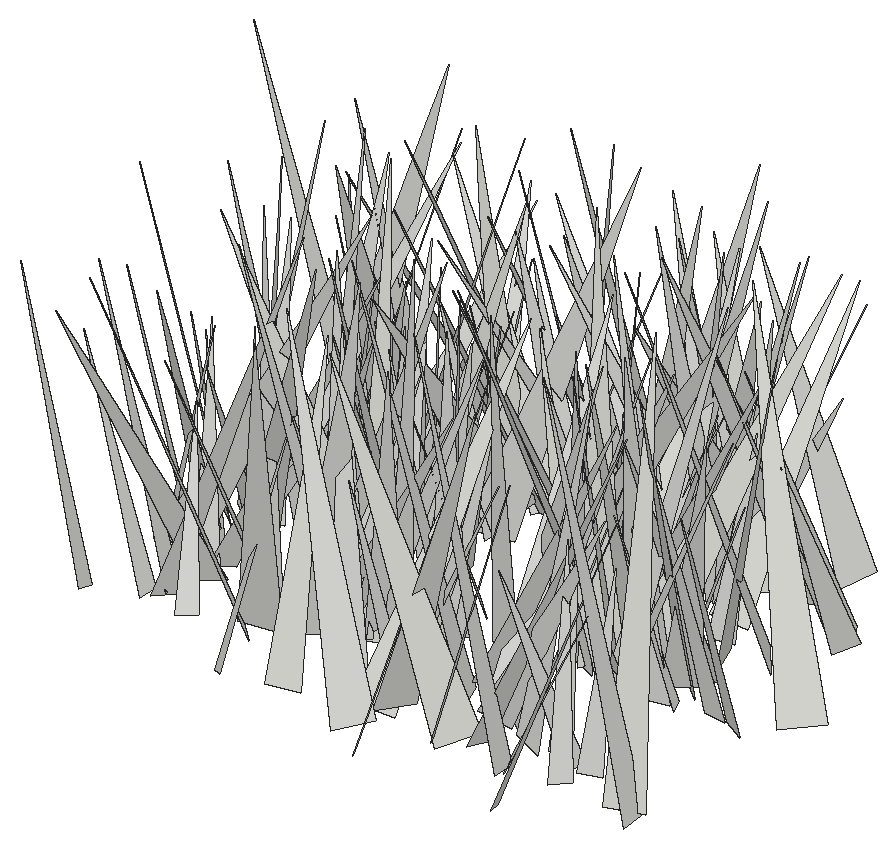
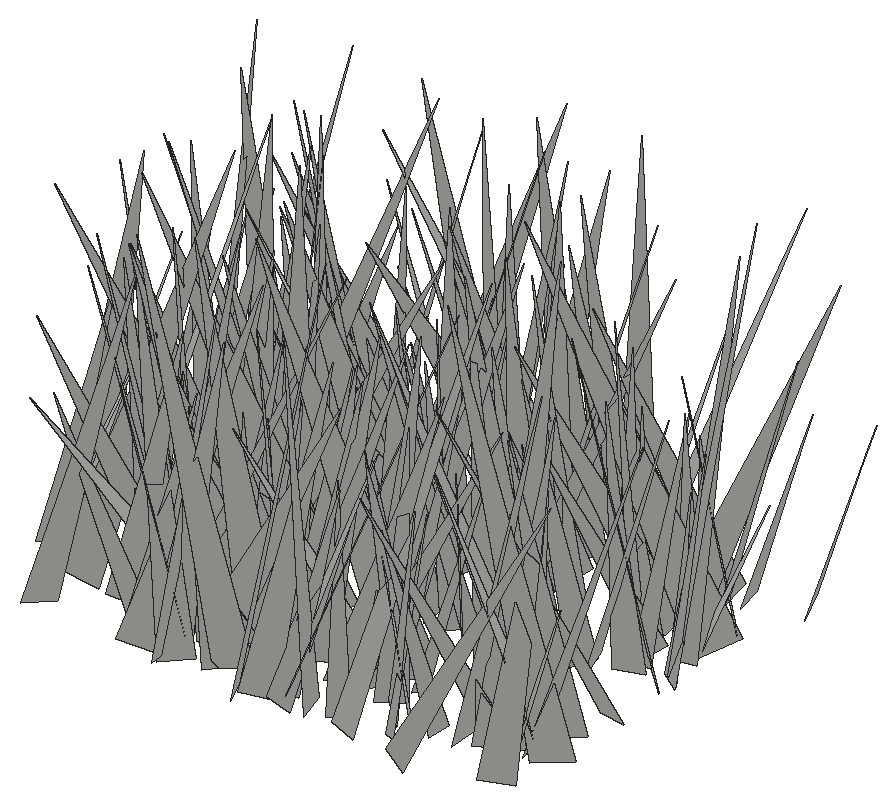
# SketchUp Ruby script. Lengths in inches.
U = 1.inch
M = Sketchup.active_model
def pt(a) = Geom::Point3d.new(a.map { |v| v * U })
def face(e, loops, mat)
  f = e.add_face(loops[0].map { |a| pt(a) })
  loops[1..].each { |l| e.add_face(l.map { |a| pt(a) }).erase! }
  f.material = f.back_material = mat if mat
  f
end
# faces: each face lists its corners as indices into pts; further lists are holes
def faces(e, pts, list, mat = nil) = list.each { |f| face(e, (f[0].is_a?(Array) ? f : [f]).map { |l| l.map { |i| pts[i] } }, mat) }
# xy, xz, yz: faces in a plane at the given z, y or x. An outline is a flat list of corners, or four numbers for a rectangle; further outlines are holes
def ring(l) = l.size == 4 ? [[l[0], l[1]], [l[2], l[1]], [l[2], l[3]], [l[0], l[3]]] : l.each_slice(2).to_a
def flat(e, list, mat, &to3) = list.each { |f| face(e, (f[0].is_a?(Array) ? f : [f]).map { |l| ring(l).map { |u, v| to3.(u, v) } }, mat) }
def xy(e, z, list, mat = nil) = flat(e, list, mat) { |x, y| [x, y, z] }
def xz(e, y, list, mat = nil) = flat(e, list, mat) { |x, z| [x, y, z] }
def yz(e, x, list, mat = nil) = flat(e, list, mat) { |y, z| [x, y, z] }
def lines(e, pts, list) = list.each { |a, b| e.add_line(pt(pts[a]), pt(pts[b])) }
# prism: a flat outline (further loops are holes) pulled along v
def prism(e, loops, v, mat = nil)
  f = face(e, loops, mat); d = Geom::Vector3d.new(v.map { |x| x * U })
  f.pushpull(f.normal.samedirection?(d) ? d.length : -d.length)
end
def box(e, o, s, mat = nil) = prism(e, [[o, [o[0] + s[0], o[1], o[2]], [o[0] + s[0], o[1] + s[1], o[2]], [o[0], o[1] + s[1], o[2]]]], [0, 0, s[2]], mat)
def at(x, y, z, deg = 0) = Geom::Transformation.translation(pt([x, y, z])) * Geom::Transformation.rotation(ORIGIN, Z_AXIS, deg.degrees)
def axes(o, x, y, z) = Geom::Transformation.new([*x, 0, *y, 0, *z, 0, *pt(o).to_a, 1])
def part(name) = M.definitions.add(name)
# library, detail: a bought-in or finely detailed component or shape, given as its bounding box
def library(name, o, s) = part(name).tap { |d| box(d.entities, o, s) }
def detail(e, o, s) = box(e.add_group.entities, o, s)
def put(e, d, t, mat = nil) = e.add_instance(d, t).tap { |i| i.material = mat if mat }
def group(e, t, mat = nil) = e.add_group.tap { |g| g.transformation = t; g.material = mat if mat }.entities
root = M.entities
c1 = part("fur_instance\#9")
p = [[0.8125,0,1.79],[0.67,-0.02,1.48],[0,-0.11,0],[0,0.11,0]]
faces(c1.entities,p,[[0,1,2,3]])
put(root,c1,axes([472.84,42.34,-21.86],[-5.74656,4.30747,2.03787],[4.75581,5.38477,2.02895],[0.29923,-2.86007,6.88916]))
put(root,c1,axes([476.6,39.5625,-21.86],[4.68389,2.5085,0.46697],[2.25732,-4.52881,1.68637],[-1.1896,1.28326,5.03861]))
put(root,c1,axes([475.14,42.1,-21.86],[3.88446,1.51086,0.00017],[1.46105,-3.75628,-1.06181],[0.38475,-0.98965,4.03042]))
put(root,c1,axes([469.49,40.97,-21.86],[-6.20404,3.776,0.73856],[3.82283,6.20814,0.37243],[0.43544,-0.70326,7.25325]))
put(root,c1,axes([469.79,42.79,-21.86],[6.355,-3.28716,0.66061],[-3.33311,-6.3472,0.48096],[-0.36352,0.73183,7.13864]))
put(root,c1,axes([462.65,43.82,-21.86],[-5.16383,-5.19186,0.43743],[-5.2089,5.15828,-0.26709],[0.11856,0.49863,7.31773]))
put(root,c1,axes([462.92,44.23,-21.86],[2.24537,-6.9608,0.71668],[-6.96969,-2.1575,0.8813],[0.62434,0.94895,7.26069]))
put(root,c1,axes([480.78,41.78,-21.86],[-7.60093,-1.69118,1.08047],[-1.85126,7.54274,-1.21718],[0.77483,1.43129,7.69108]))
put(root,c1,axes([477.04,43.34,-21.86],[0.84597,-3.78981,1.14812],[-3.67965,-1.18614,-1.20406],[-1.46323,0.79177,3.69169]))
put(root,c1,axes([471.96,42.2,-21.86],[4.69401,2.26049,0.88712],[2.32694,-4.7392,-0.23643],[-0.69438,-0.60059,5.20458]))
put(root,c1,axes([475.27,41.71,-21.86],[-7.26619,-2.16018,0.91047],[-2.32448,7.02333,-1.88745],[0.30351,2.07347,7.34176]))
put(root,c1,axes([470.62,39.66,-21.86],[6.47169,4.71895,0.84374],[4.29058,-6.33416,2.51645],[-2.13805,1.57262,7.60387]))
put(root,c1,axes([463.71,40.98,-21.86],[2.88186,3.44939,0.31018],[3.15851,-2.7832,1.60537],[-1.42067,0.8094,4.19835]))
put(root,c1,axes([477.31,42.17,-21.86],[-3.68366,1.92684,0.76086],[1.83141,3.75443,-0.64122],[0.96827,0.22919,4.10742]))
put(root,c1,axes([466.07,41.49,-21.86],[-1.14776,6.0133,0.84328],[6.0716,1.14805,0.07727],[0.08148,-0.84289,6.12137]))
put(root,c1,axes([459.61,45.74,-21.86],[0.6668,-6.36542,0.43774],[-6.10772,-0.7641,-1.80742],[-1.84553,0.22889,6.13974]))
put(root,c1,axes([477.73,43.23,-21.86],[-1.6026,3.32948,1.45838],[3.48573,1.8596,-0.41502],[1.03054,-1.11225,3.67172]))
put(root,c1,axes([472.91,44.2,-21.86],[2.62599,-5.06265,0.78885],[-4.77605,-2.09765,2.43674],[1.85526,1.76578,5.15641]))
put(root,c1,axes([468.62,44.36,-21.86],[-3.79793,-0.43925,1.06155],[-0.29859,3.91782,0.55288],[1.10936,-0.44932,3.78306]))
put(root,c1,axes([456.67,42.78,-21.86],[-5.41168,-1.42657,0.35166],[-1.45652,5.03228,-1.99993],[-0.1932,2.0214,5.22701]))
put(root,c1,axes([458.56,43.73,-21.86],[-4.63616,-0.58897,0.33378],[-0.62989,4.59941,-0.63319],[0.24806,0.67142,4.63033]))
put(root,c1,axes([475.93,43.92,-21.86],[-2.42915,2.39744,1.43013],[2.49267,2.71628,-0.31959],[1.25681,-0.75355,3.39799]))
put(root,c1,axes([473.52,42.63,-21.86],[6.28882,0.29269,0.74734],[0.08478,-6.11246,1.68051],[-0.79813,1.65699,6.06719]))
put(root,c1,axes([464.66,45.01,-21.86],[5.72788,-5.11466,1.67521],[-5.30647,-5.77538,0.51083],[-0.89854,1.50329,7.66207]))
put(root,c1,axes([466.98,43.83,-21.86],[1.5886,-5.12639,3.23902],[-5.9044,-2.07062,-0.3813],[-1.38174,2.95423,5.35333]))
put(root,c1,axes([460.48,43.38,-21.86],[-2.65941,2.49787,0.36396],[2.46932,2.68404,-0.37765],[0.52369,0.0288,3.62894]))
put(root,c1,axes([474.83,43.53,-21.86],[2.70818,5.99392,1.73773],[6.22026,-2.74585,-0.22279],[-0.5051,-1.67756,6.57356]))
put(root,c1,axes([480.12,42.08,-21.86],[-0.32528,8.12923,0.88129],[8.06717,0.17507,1.36272],[-1.33486,-0.92294,8.0208]))
put(root,c1,axes([461.41,46.38,-21.86],[-3.58338,-3.97137,0.418],[-3.89573,3.60001,0.80641],[0.87736,-0.23507,5.28792]))
put(root,c1,axes([466.74,46.08,-21.86],[2.07468,-5.92746,1.15005],[-6.03286,-1.98482,0.6533],[0.24901,1.299,6.24598]))
put(root,c1,axes([468.7,44.78,-21.86],[3.8277,2.64651,0.3376],[2.6435,-3.68235,-1.10521],[0.36045,-1.09797,4.52038]))
put(root,c1,axes([458.97,44.52,-21.86],[-5.59376,-1.56322,0.76508],[-1.67452,5.53596,-0.93185],[0.47433,1.10847,5.73284]))
put(root,c1,axes([471.3,44.89,-21.86],[-7.24522,-3.15461,1.03201],[-3.28219,7.17812,-1.10079],[0.49381,1.42581,7.82516]))
put(root,c1,axes([465.98,45.17,-21.86],[-6.93543,-2.32629,0.88421],[-2.41004,6.93097,-0.66862],[0.62063,0.91853,7.28456]))
put(root,c1,axes([467.8,45.45,-21.86],[-2.07525,-6.86081,3.30693],[-7.48887,2.46229,0.40886],[1.38687,3.02978,7.15613]))
put(root,c1,axes([464.85,45.8,-21.86],[4.53332,-3.78068,0.06575],[-3.6354,-4.32956,1.69931],[1.04008,1.34544,5.65304]))
put(root,c1,axes([457.58,48.37,-21.86],[-1.80775,-6.68688,0.47497],[-6.40102,1.86794,1.93536],[1.9917,-0.06601,6.65106]))
put(root,c1,axes([469.32,42.23,-21.86],[-4.67484,5.38464,0.57126],[4.73589,4.43174,-3.01759],[2.62527,1.59378,6.46085]))
put(root,c1,axes([457.66,45.52,-21.86],[3.51843,3.11531,1.14482],[3.25687,-3.56198,-0.31656],[-0.63919,-1.00114,4.68874]))
put(root,c1,axes([476.61,46.13,-21.86],[-3.5972,0.42819,0.55364],[0.48536,3.61469,0.35791],[0.50428,-0.42464,3.60487]))
put(root,c1,axes([459.07,43.98,-21.86],[6.5419,0.41912,1.71437],[-0.23349,-6.31856,2.43568],[-1.74935,2.41069,6.08602]))
put(root,c1,axes([464.67,46.52,-21.86],[-4.98307,4.13485,3.06586],[4.6284,5.46651,0.15019],[2.25263,-2.08511,6.47344]))
put(root,c1,axes([475.45,48.02,-21.86],[-4.28269,-7.03673,0.88853],[-7.06243,4.13524,-1.29164],[-0.65353,1.42504,8.13564]))
put(root,c1,axes([465.53,44.9375,-21.86],[1.79121,4.66243,0.42191],[4.67903,-1.79759,0.00003],[-0.15134,-0.39383,4.99466]))
put(root,c1,axes([465.98,46.38,-21.86],[3.63408,5.21962,1.38175],[5.32326,-3.18476,-1.96987],[0.90365,-2.23003,6.04736]))
put(root,c1,axes([465.93,48.52,-21.86],[-3.21608,-6.87634,1.40534],[-6.91778,3.36666,0.64196],[1.18463,0.99184,7.56406]))
put(root,c1,axes([461.64,45.5,-21.86],[-4.54245,-0.30979,1.16713],[-0.64985,4.4561,-1.34644],[1.01777,1.46262,4.34936]))
put(root,c1,axes([459.35,48.45,-21.86],[7.07591,-3.11018,0.05148],[-3.09924,-7.06002,-0.5432],[-0.26559,-0.47663,7.71016]))
put(root,c1,axes([459.13,46.125,-21.86],[-1.17354,4.22506,1.16991],[4.38332,1.15287,0.2334],[0.0799,-1.19029,4.3788]))
put(root,c1,axes([471.13,46.07,-21.86],[5.6454,-1.61471,0.55375],[-1.70236,-5.46688,1.41409],[-0.12614,1.5134,5.69896]))
put(root,c1,axes([470.58,48.1,-21.86],[5.01746,5.30698,2.27397],[5.71554,-4.13917,-2.95123],[0.81705,-3.63499,6.68051]))
put(root,c1,axes([468.27,47.51,-21.86],[4.61817,-3.87726,2.02523],[-4.05143,-4.90172,-0.14567],[-1.64942,1.18414,6.02822]))
put(root,c1,axes([476.12,50.36,-21.86],[-3.7888,-7.35051,1.42507],[-6.56657,4.02946,3.32556],[3.59735,-0.38635,7.57137]))
put(root,c1,axes([473.87,44.2,-21.86],[4.6203,4.92142,0.32663],[4.69042,-4.52255,1.79463],[-1.52544,1.00021,6.50745]))
put(root,c1,axes([475.52,47.16,-21.86],[5.31801,3.62577,0.57345],[3.65614,-5.14142,-1.39812],[0.32822,-1.47507,6.28273]))
put(root,c1,axes([457.16,49.66,-21.86],[-4.90749,-6.3294,1.61985],[-6.13533,5.16095,1.5783],[2.24565,0.26836,7.85199]))
put(root,c1,axes([479.5,48.63,-21.86],[-1.94034,-4.30134,0.80925],[-4.30819,2.03312,0.47669],[0.77193,0.53502,4.69459]))
put(root,c1,axes([463.92,46.3,-21.86],[6.69974,-1.69034,1.74311],[-2.11177,-6.58131,1.73465],[-1.19837,2.1474,6.68841]))
put(root,c1,axes([472.65,48.95,-21.86],[-1.45623,-6.82166,1.9418],[-6.84757,1.86878,1.42991],[1.84835,1.54881,6.82723]))
put(root,c1,axes([462.31,45.52,-21.86],[-6.71472,0.14595,1.05093],[-0.21339,6.41005,-2.25365],[1.03933,2.25902,6.32691]))
put(root,c1,axes([464.58,48.4,-21.86],[-7.38136,0.22251,0.33251],[0.26326,7.32737,0.9407],[0.30128,-0.95116,7.32455]))
put(root,c1,axes([458.59,49.45,-21.86],[-0.44013,-4.40012,0.04518],[-4.35564,0.44209,0.62427],[0.62566,-0.01764,4.37779]))
put(root,c1,axes([470.26,48.11,-21.86],[-1.72933,-6.01967,2.37326],[-6.41752,1.90965,0.16749],[0.82719,2.23073,6.26091]))
put(root,c1,axes([457.25,46.99,-21.86],[6.5519,-4.81181,0.9912],[-4.80718,-5.93833,2.94799],[1.01342,2.94042,7.57563]))
put(root,c1,axes([474.39,48.88,-21.86],[4.90048,2.76624,3.25214],[3.64641,-5.28694,-0.99757],[-2.22086,-2.5767,5.5382]))
put(root,c1,axes([466.49,46.08,-21.86],[-5.1152,1.11044,1.16629],[0.73583,5.06638,-1.59654],[1.43244,1.36283,4.98492]))
put(root,c1,axes([468.25,47.1,-21.86],[1.29664,4.3065,0.97913],[4.41517,-1.23995,-0.39328],[0.1042,-1.05001,4.48024]))
put(root,c1,axes([467.59,47.84,-21.86],[-4.97388,0.03891,0.99351],[0.0174,5.07103,-0.11152],[0.99411,0.10595,4.97278]))
put(root,c1,axes([467.87,49.89,-21.86],[-3.10311,-4.08719,0.56583],[-3.96021,3.14894,1.02739],[1.15846,-0.18348,5.02781]))
put(root,c1,axes([478.54,48.85,-21.86],[-1.41742,-4.71426,1.18858],[-4.85717,1.31918,-0.56008],[-0.21176,1.29675,4.89077]))
put(root,c1,axes([472.74,47.15,-21.86],[3.10796,2.24348,0.34109],[2.21254,-3.12436,0.38987],[-0.50422,0.11876,3.81322]))
put(root,c1,axes([474.71,49.58,-21.86],[-2.15861,-6.19615,1.53511],[-6.31129,2.3146,0.46773],[0.95736,1.28794,6.5447]))
put(root,c1,axes([457.85,47.08,-21.86],[-4.45593,-2.02584,0.38216],[-1.95722,3.87117,-2.29973],[-0.64758,2.23951,4.32095]))
put(root,c1,axes([463.16,51.05,-21.86],[-1.84691,-6.18778,0.26193],[-5.9057,1.84189,1.87043],[1.86547,-0.29517,6.18071]))
put(root,c1,axes([472.33,45.86,-21.86],[-2.04424,6.85145,0.72305],[6.79433,2.1298,-0.97223],[1.1412,-0.40704,7.08351]))
put(root,c1,axes([476.36,49.76,-21.86],[4.15858,-4.6502,0.45845],[-4.67236,-4.14601,0.32855],[-0.05962,0.56087,6.22978]))
put(root,c1,axes([477.08,48.64,-21.86],[-3.24657,-1.58505,0.39086],[-1.61743,3.24104,-0.29141],[0.22149,0.43432,3.60107]))
put(root,c1,axes([458.31,47.83,-21.86],[1.10778,3.32388,1.25845],[3.28018,-1.46364,0.97838],[-1.36832,-0.8177,3.36424]))
put(root,c1,axes([466.34,45.76,-21.86],[0.27633,8.1596,0.76138],[7.93766,-0.45592,2.00518],[-2.0377,-0.66947,7.91421]))
put(root,c1,axes([459.36,46.67,-21.86],[6.04009,-0.71684,0.90558],[-1.00409,-5.64184,2.23115],[-0.57074,2.3393,5.65849]))
put(root,c1,axes([467.11,48.35,-21.86],[3.97041,-1.42005,1.05601],[-1.57618,-4.01704,0.5243],[-0.80459,0.86179,4.18399]))
put(root,c1,axes([474.36,50.43,-21.86],[3.11086,-6.46121,1.0779],[-6.53922,-3.13316,0.09147],[-0.38422,1.01124,7.17051]))
put(root,c1,axes([476.76,50.81,-21.86],[-0.49515,-5.81147,0.35136],[-5.82208,0.49376,-0.03799],[-0.0081,0.35331,5.8324]))
put(root,c1,axes([476.39,48.49,-21.86],[-0.90978,-4.59674,2.27002],[-5.08569,0.51819,-0.98893],[-0.64715,2.39002,4.58036]))
put(root,c1,axes([458.76,48.4,-21.86],[3.29977,-2.51906,0.3221],[-2.3698,-2.86445,1.87534],[0.91296,1.66948,3.70368]))
put(root,c1,axes([457.1,49.63,-21.86],[-2.14945,-3.42966,1.0737],[-3.50191,2.27993,0.27214],[0.80747,0.75821,4.03839]))
put(root,c1,axes([465.57,47.7,-21.86],[-4.06355,5.05875,1.67662],[5.05755,4.32523,-0.79246],[1.68023,-0.78477,6.44014]))
put(root,c1,axes([475.32,47.42,-21.86],[2.96798,6.81466,1.03357],[6.887,-2.97737,-0.1458],[-0.27767,-1.00619,7.4315]))
put(root,c1,axes([463.35,46.91,-21.86],[2.8075,7.47142,1.47372],[7.21104,-3.11318,2.04573],[-2.44844,-0.60171,7.71486]))
put(root,c1,axes([459.7,48.22,-21.86],[-6.13991,-1.94187,2.86824],[-2.65031,6.39227,-1.34568],[2.23013,2.25037,6.2975]))
put(root,c1,axes([460.17,50.5,-21.86],[4.67852,-1.7119,0.20248],[-1.71617,-4.68064,0.08066],[-0.16239,0.14538,4.98123]))
put(root,c1,axes([473.03,50.95,-21.86],[-3.56669,-5.90918,0.59479],[-5.71236,3.22345,-2.22975],[-1.62517,1.63841,6.53207]))
put(root,c1,axes([466.43,50.08,-21.86],[4.38059,2.58911,2.20412],[2.75267,-4.81057,0.18002],[-1.99611,-0.9519,5.08534]))
put(root,c1,axes([473.29,49.41,-21.86],[-7.16118,3.19135,1.99245],[3.1192,7.43157,-0.69239],[2.1036,-0.15533,7.80947]))
put(root,c1,axes([458.63,49.99,-21.86],[-1.35199,5.16754,1.66066],[5.39955,1.4549,-0.13134],[0.55327,-1.57128,5.33986]))
put(root,c1,axes([466.04,51.18,-21.86],[5.32416,0.8497,1.29821],[1.01973,-5.41351,-0.63884],[-1.1694,-0.85204,5.35356]))
put(root,c1,axes([462.61,52.26,-21.86],[4.90607,-3.46037,0.24315],[-3.44997,-4.91123,-0.28332],[-0.36191,-0.09172,5.99695]))
put(root,c1,axes([464.875,51.35,-21.86],[2.7967,-3.72992,1.22325],[-3.91864,-2.74089,0.60164],[-0.23004,1.34365,4.62297]))
put(root,c1,axes([477.53,53.06,-21.86],[-6.16047,-5.25921,0.96963],[-5.25018,6.22911,0.42963],[1.01736,0.29959,8.08864]))
put(root,c1,axes([459.83,50.47,-21.86],[-6.22819,-1.34042,0.61243],[-1.44458,6.07908,-1.38568],[0.29149,1.48668,6.21828]))
put(root,c1,axes([469.69,54.03,-21.86],[-1.30326,-6.4856,0.41929],[-6.05179,1.36694,2.33336],[2.36951,-0.07596,6.19006]))
put(root,c1,axes([464.85,55.5,-21.86],[6.08431,-4.17162,0.61258],[-3.3903,-5.47976,-3.64343],[-2.50671,-2.71408,6.41457]))
put(root,c1,axes([481.18,50.18,-21.86],[-5.24663,5.623,0.95369],[5.70188,5.20042,0.70642],[0.12741,-1.17997,7.65808]))
put(root,c1,axes([457.58,49.91,-21.86],[4.64173,5.41011,1.53464],[5.42173,-4.8336,0.64123],[-1.49305,-0.73288,7.09956]))
put(root,c1,axes([474.84,52.28,-21.86],[3.70621,1.73352,0.50221],[1.78343,-3.34171,-1.62653],[0.27688,-1.67963,3.75439]))
put(root,c1,axes([461.38,50.32,-21.86],[-4.14484,-0.82966,2.07391],[-1.4546,4.32013,-1.17886],[1.69516,1.67847,4.05935]))
put(root,c1,axes([476.33,52.06,-21.86],[6.26752,1.77798,1.53658],[2.00319,-6.33057,-0.84565],[-1.22862,-1.25168,6.45971]))
put(root,c1,axes([469.45,52.57,-21.86],[3.81653,-4.78014,0.36891],[-4.62204,-3.54318,1.90641],[1.2738,1.46558,5.81217]))
put(root,c1,axes([470.42,51.53,-21.86],[-1.43576,4.62376,1.24523],[4.74317,1.1948,1.0324],[-0.65727,-1.47798,4.73019]))
put(root,c1,axes([472.49,52.375,-21.86],[5.56558,-2.4926,0.3103],[-2.49513,-5.39934,1.38077],[0.28926,1.38533,5.93988]))
put(root,c1,axes([469.34,54.14,-21.86],[-3.93498,0.71077,2.15609],[1.47172,4.08376,1.33974],[1.72857,-1.85895,3.76754]))
put(root,c1,axes([468.71,53.08,-21.86],[6.17977,-5.38552,0.13557],[-5.06059,-5.73249,2.95646],[1.84733,2.31224,7.64543]))
put(root,c1,axes([463.34,52.11,-21.86],[2.20928,6.37096,1.50715],[6.50914,-1.9672,-1.22586],[0.70121,-1.81177,6.63078]))
put(root,c1,axes([470.39,54.03,-21.86],[0.55845,-3.67703,0.59896],[-3.72525,-0.55803,0.04757],[-0.0423,0.59936,3.71889]))
put(root,c1,axes([475.46,53.04,-21.86],[-1.45732,3.49071,1.72371],[3.67662,1.83923,-0.61623],[1.28012,-1.30851,3.73217]))
put(root,c1,axes([474.17,51.19,-21.86],[-6.70082,0.16595,0.10129],[0.12128,6.29761,-2.29436],[0.15195,2.29157,6.29797]))
put(root,c1,axes([458.85,56.79,-21.86],[7.11754,-4.23376,0.53848],[-3.90576,-6.88369,-2.49681],[-1.7204,-1.88792,7.89621]))
put(root,c1,axes([473.84,51.23,-21.86],[-0.75445,7.6495,1.46212],[7.18414,1.25072,-2.83648],[3.00677,-1.06897,7.14412]))
put(root,c1,axes([465.08,54.12,-21.86],[-4.43499,0.78648,1.49873],[1.10021,4.53377,0.87655],[1.28619,-1.16631,4.41807]))
put(root,c1,axes([472.4375,52.11,-21.86],[-1.23415,4.06964,0.18802],[4.01431,1.18128,0.78126],[-0.69473,-0.40381,4.18028]))
put(root,c1,axes([479.04,55.21,-21.86],[3.36953,-3.09183,0.80409],[-2.80421,-3.42236,-1.4084],[-1.53048,-0.53643,4.35081]))
put(root,c1,axes([462.41,51.5,-21.86],[6.70956,3.50603,1.11128],[3.28027,-6.75003,1.49074],[-1.66343,0.8308,7.42214]))
put(root,c1,axes([478.33,55.42,-21.86],[-4.87517,-3.87645,0.62854],[-3.83008,4.91477,0.6039],[0.86741,-0.08574,6.19915]))
put(root,c1,axes([460.75,54.97,-21.86],[3.22144,-2.0672,0.86258],[-1.86043,-3.31076,-0.98626],[-1.24746,-0.40075,3.69841]))
put(root,c1,axes([472.48,52.91,-21.86],[3.75823,0.40452,0.85087],[0.18545,-3.74836,0.96295],[-0.9237,0.89332,3.65522]))
put(root,c1,axes([472.27,53.09,-21.86],[-3.57041,1.71359,0.7726],[1.61509,3.64514,-0.62093],[0.96166,0.24019,3.91135]))
put(root,c1,axes([476.71,56.74,-21.66],[0.82289,-7.98079,0.80674],[-7.83354,-0.97405,-1.64552],[-1.72608,0.61581,7.85254]))
put(root,c1,axes([463.17,55.43,-21.86],[-3.68775,-0.43694,1.2324],[0.03671,3.65173,1.40455],[1.30705,-1.33536,3.43768]))
put(root,c1,axes([470.85,53.98,-21.86],[3.29309,2.39527,0.08068],[2.3726,-3.23886,-0.68467],[0.3385,-0.60058,4.0141]))
put(root,c1,axes([472.77,56.27,-21.66],[-6.88482,-1.0416,0.48285],[-0.90858,6.73783,1.57954],[0.70182,-1.49517,6.78165]))
put(root,c1,axes([459.96,53.21,-21.86],[-5.24858,-0.93793,1.2858],[-1.33069,5.01688,-1.77222],[0.87308,2.00792,5.02857]))
put(root,c1,axes([464.95,53.86,-21.86],[5.54256,-5.39998,2.31392],[-5.86744,-4.92827,2.55329],[0.29519,3.43313,7.30483]))
put(root,c1,axes([468.37,54.75,-21.86],[-4.97411,1.9133,1.24146],[2.05101,5.05519,0.42681],[0.99764,-0.85328,5.31228]))
put(root,c1,axes([466.625,58.12,-21.86],[-5.86145,-3.99032,0.23805],[-3.68658,5.55942,2.41617],[1.54546,-1.87245,6.66644]))
put(root,c1,axes([467.24,55.92,-21.86],[3.86572,-4.28586,2.24353],[-4.19582,-4.39988,-1.17556],[-2.40771,0.7863,5.6507]))
put(root,c1,axes([473.4375,55.6,-21.86],[-6.84332,-0.22544,2.15666],[-0.013,7.14388,0.70553],[2.16837,-0.66867,6.81058]))
put(root,c1,axes([457.0625,52.83,-21.86],[2.4491,6.4359,0.09226],[6.32974,-2.3903,-1.28384],[1.16776,-0.54137,6.7654]))
put(root,c1,axes([470.93,52.76,-21.86],[-1.68385,4.77561,0.18208],[4.53538,1.65768,-1.53538],[1.50664,0.34725,4.82539]))
put(root,c1,axes([461.58,55.07,-21.86],[3.09242,2.58599,1.68004],[2.84079,-3.31463,-0.12697],[-1.19992,-1.18273,4.02918]))
put(root,c1,axes([458.24,56.45,-21.86],[-0.42992,-4.68733,0.89248],[-4.33891,0.75688,1.88505],[1.98531,0.63912,4.31306]))
put(root,c1,axes([474.08,55.64,-21.86],[4.94298,-3.20176,1.42299],[-3.34359,-5.04595,0.26096],[-1.0472,0.99819,5.88356]))
put(root,c1,axes([465.36,56.08,-21.86],[-3.41079,-4.86692,0.40111],[-4.72199,3.16213,-1.78467],[-1.24525,1.33989,5.66881]))
put(root,c1,axes([473.08,52.46,-21.86],[-5.5806,3.5391,0.90465],[3.04631,5.42049,-2.4135],[2.01583,1.60617,6.15169]))
put(root,c1,axes([457.4,54.7,-21.86],[2.82826,-4.43632,2.67471],[-5.15951,-2.68482,1.00262],[-0.46309,2.81866,5.16476]))
put(root,c1,axes([478.62,56.17,-21.86],[-4.47388,-2.50611,0.21033],[-2.51468,4.46372,-0.30343],[0.03476,0.36756,5.119]))
put(root,c1,axes([468.42,55.99,-21.86],[-4.16703,-2.76107,2.92288],[-2.78486,5.0182,0.77013],[2.90022,0.85149,4.93909]))
put(root,c1,axes([472.5,58.83,-21.86],[3.62515,-5.36286,0.15908],[-5.03579,-3.46731,-2.13211],[-1.85105,-1.06996,6.11196]))
put(root,c1,axes([469.62,55.74,-21.86],[6.54433,-2.87567,1.841],[-3.10892,-6.66403,0.64215],[-1.41189,1.3447,7.11937]))
put(root,c1,axes([473.12,55.3,-21.86],[3.79421,5.57197,1.64798],[5.81056,-3.63804,-1.07735],[0.00109,-1.96889,6.65448]))
put(root,c1,axes([463.58,59.05,-21.86],[-3.81436,-7.20009,0.2192],[-7.12697,3.80817,1.069],[1.0467,-0.30859,8.07762]))
put(root,c1,axes([464.49,55.94,-21.86],[-6.37075,2.32719,2.17346],[2.54476,6.64308,0.34616],[1.91413,-1.08621,6.77365]))
put(root,c1,axes([471.48,54.61,-21.86],[7.05742,-1.09775,2.22467],[-1.64487,-7.09246,1.71837],[-1.85705,2.1103,6.93249]))
put(root,c1,axes([467.2,53.7,-21.86],[4.59925,2.87418,0.36346],[2.61006,-4.40682,1.82035],[-1.25721,1.36572,5.10885]))
put(root,c1,axes([457.16,58.87,-21.66],[4.65411,-4.15615,0.09318],[-4.0063,-4.52139,-1.56511],[-1.10988,-1.10744,6.04026]))
put(root,c1,axes([470.58,57.67,-21.66],[4.65665,4.64477,2.8893],[5.46904,-4.02795,-2.33914],[-0.10763,-3.71592,6.14709]))
put(root,c1,axes([460.09,56.95,-21.86],[-6.59248,-1.12335,1.64682],[-1.04061,6.79216,0.46743],[1.70031,-0.1986,6.67115]))
put(root,c1,axes([458.04,55.73,-21.86],[-7.51977,-1.08655,0.44758],[-1.14316,7.43533,-1.15625],[0.27218,1.20961,7.50937]))
put(root,c1,axes([456.54,56.65,-21.66],[0.11593,7.32982,3.76994],[7.80213,1.11829,-2.4142],[2.6581,-3.60212,6.9218]))
put(root,c1,axes([465.49,56.51,-21.86],[-4.72001,4.32069,1.36462],[4.52973,4.45158,1.57294],[-0.11027,-2.07946,6.20264]))
put(root,c1,axes([463.49,56.55,-21.86],[2.88206,-3.90926,2.29022],[-4.22914,-3.29495,-0.30223],[-1.62535,1.64154,4.8474]))
put(root,c1,axes([466.43,58.97,-21.86],[-1.51656,-6.50321,0.08888],[-6.50028,1.51258,-0.24097],[-0.21452,0.14123,6.67335]))
put(root,c1,axes([469.66,56.38,-21.86],[3.69637,0.13401,0.11411],[0.12786,-3.69317,0.19555],[-0.12096,0.19138,3.69362]))
put(root,c1,axes([474.82,54.26,-21.86],[-1.93845,6.02083,0.54238],[5.77969,2.01278,-1.68701],[1.77192,0.02133,6.09606]))
put(root,c1,axes([472.61,56.125,-21.86],[4.17066,5.06918,1.33611],[5.23853,-4.09478,-0.81653],[-0.19883,-1.55319,6.51339]))
put(root,c1,axes([463.98,54.93,-21.86],[-3.2921,4.67046,0.35788],[4.62081,3.30978,-0.68745],[0.76768,0.10645,5.67261]))
put(root,c1,axes([470.97,56.27,-21.86],[-3.29072,5.65648,0.59206],[5.32719,2.82602,2.60955],[-1.99181,-1.7869,6.00123]))
put(root,c1,axes([470.85,58.76,-21.86],[1.7793,-6.50243,0.4842],[-6.28195,-1.575,1.93351],[1.74732,0.95904,6.45825]))
put(root,c1,axes([462.09,58.41,-21.86],[-2.01295,-3.23513,0.63988],[-3.06607,2.112,1.03257],[1.21439,-0.03018,3.66768]))
put(root,c1,axes([469.43,58.34,-21.86],[2.01974,-4.62687,0.27657],[-4.52399,-1.90214,1.21619],[1.00891,0.73329,4.89981]))
put(root,c1,axes([461.68,57.7,-21.86],[4.05743,2.55482,1.17911],[2.80714,-3.81746,-1.3882],[-0.19333,-1.81108,4.58942]))
put(root,c1,axes([473.25,57.9375,-21.86],[3.41803,-2.18502,2.15563],[-1.95303,-4.03718,-0.99543],[-2.36786,0.1758,3.93273]))
put(root,c1,axes([464.22,58.4375,-21.86],[1.68223,-3.64936,0.16027],[-3.63941,-1.65928,0.41825],[0.31341,0.31999,3.9966]))
put(root,c1,axes([467.22,59.01,-21.86],[2.93992,-5.13493,1.13143],[-5.01799,-3.12719,-1.15379],[-1.5708,0.37938,5.8034]))
put(root,c1,axes([458.1,56.64,-21.66],[-3.16034,-1.96863,0.75138],[-2.10046,2.8354,-1.40585],[-0.16774,1.5852,3.44773]))
put(root,c1,axes([474.65,56.7,-21.86],[-2.33709,5.71521,1.48586],[5.84354,2.00796,1.46781],[-0.85111,-1.90732,5.99759]))
put(root,c1,axes([461.02,57.1,-21.86],[3.85375,-0.57416,0.66525],[-0.65849,-3.86826,0.47595],[-0.58191,0.57487,3.8671]))
put(root,c1,axes([466.5625,58.24,-21.86],[0.87067,-3.63818,0.96208],[-3.64876,-1.05785,-0.69825],[-0.92116,0.75142,3.67517]))
put(root,c1,axes([457.52,55.85,-21.86],[5.06961,3.19969,0.78256],[3.08145,-5.11429,0.94868],[-1.16407,0.39664,5.91937]))
put(root,c1,axes([470.76,58.24,-21.86],[3.57739,2.98141,0.96801],[3.07785,-3.06266,-1.94177],[0.59384,-2.08684,4.23274]))
put(root,c1,axes([471.41,58.96,-21.86],[-5.69321,-2.11736,2.09192],[-1.78965,6.04293,1.24584],[2.37833,-0.52131,5.94506]))
put(root,c1,axes([474.07,54.41,-21.86],[4.84887,3.21318,0.05137],[2.84684,-4.33809,2.62966],[-1.49084,2.16682,5.18854]))
put(root,c1,axes([467.72,59.54,-21.66],[-6.44031,-4.10602,1.97316],[-3.85542,6.73281,1.42663],[2.42663,-0.20036,7.50344]))
put(root,c1,axes([459.3,56.11,-21.86],[0.04423,5.29855,0.55334],[5.02486,0.14232,-1.76445],[1.76963,-0.53655,4.99632]))
put(root,c1,axes([476.65,58.78,-21.66],[-6.00437,2.1113,1.91932],[2.55574,5.96789,1.43049],[1.26869,-2.0299,6.20191]))
put(root,c1,axes([467.47,57.03,-21.86],[-5.24793,-3.08562,0.82091],[-3.15493,4.76816,-2.24651],[-0.49124,2.34081,5.65818]))
put(root,c1,axes([472.07,57.47,-21.86],[-2.9661,5.6248,1.68099],[5.86235,2.73802,1.18234],[-0.31135,-2.03143,6.24805]))
put(root,c1,axes([472.62,58.17,-21.66],[1.91277,-3.82749,0.78831],[-3.61325,-1.39793,1.9799],[1.48846,1.5251,3.7932]))
put(root,c1,axes([460.96,59.55,-21.86],[-2.19806,-5.17129,0.07017],[-4.98418,2.09779,-1.52836],[-1.38027,0.66005,5.4072]))
put(root,c1,axes([468.78,58.27,-21.66],[1.45839,-7.20301,2.88114],[-7.56056,-0.66269,2.17028],[1.73849,3.16049,7.02141]))
put(root,c1,axes([462.98,57.08,-21.86],[2.36274,4.29484,1.97791],[3.91667,-3.01643,1.87116],[-2.64906,-0.62918,4.53067]))
put(root,c1,axes([465.34,58.47,-21.86],[6.28919,2.00514,2.27548],[2.25266,-6.59596,-0.4138],[-2.03074,-1.10685,6.58812]))
